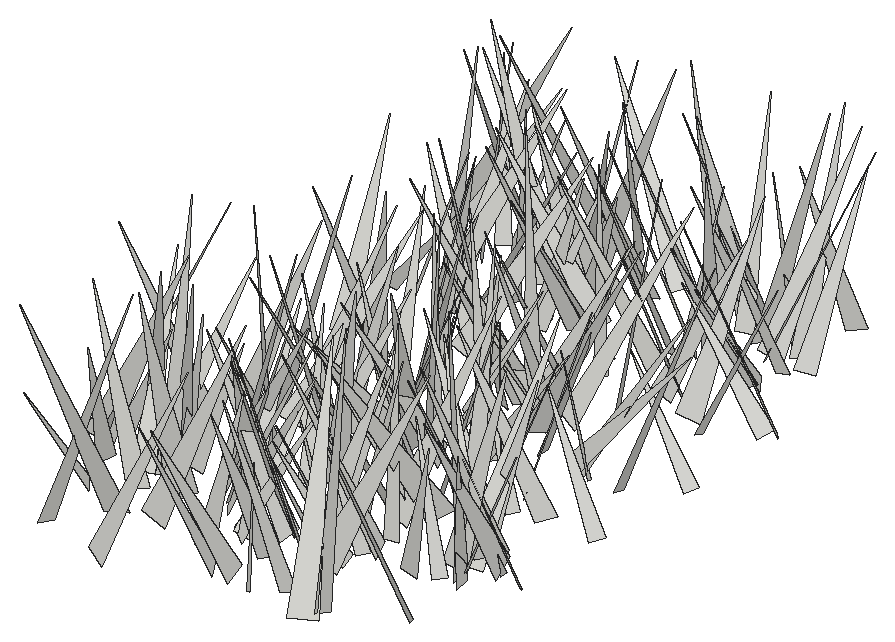
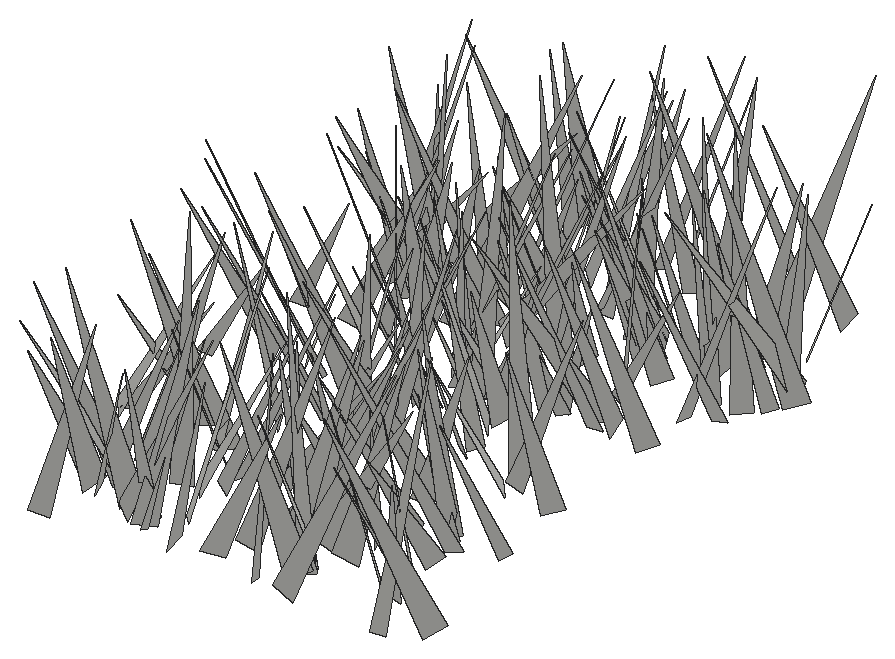
# SketchUp Ruby script. Lengths in inches.
U = 1.inch
M = Sketchup.active_model
def pt(a) = Geom::Point3d.new(a.map { |v| v * U })
def face(e, loops, mat)
  f = e.add_face(loops[0].map { |a| pt(a) })
  loops[1..].each { |l| e.add_face(l.map { |a| pt(a) }).erase! }
  f.material = f.back_material = mat if mat
  f
end
# faces: each face lists its corners as indices into pts; further lists are holes
def faces(e, pts, list, mat = nil) = list.each { |f| face(e, (f[0].is_a?(Array) ? f : [f]).map { |l| l.map { |i| pts[i] } }, mat) }
# xy, xz, yz: faces in a plane at the given z, y or x. An outline is a flat list of corners, or four numbers for a rectangle; further outlines are holes
def ring(l) = l.size == 4 ? [[l[0], l[1]], [l[2], l[1]], [l[2], l[3]], [l[0], l[3]]] : l.each_slice(2).to_a
def flat(e, list, mat, &to3) = list.each { |f| face(e, (f[0].is_a?(Array) ? f : [f]).map { |l| ring(l).map { |u, v| to3.(u, v) } }, mat) }
def xy(e, z, list, mat = nil) = flat(e, list, mat) { |x, y| [x, y, z] }
def xz(e, y, list, mat = nil) = flat(e, list, mat) { |x, z| [x, y, z] }
def yz(e, x, list, mat = nil) = flat(e, list, mat) { |y, z| [x, y, z] }
def lines(e, pts, list) = list.each { |a, b| e.add_line(pt(pts[a]), pt(pts[b])) }
# prism: a flat outline (further loops are holes) pulled along v
def prism(e, loops, v, mat = nil)
  f = face(e, loops, mat); d = Geom::Vector3d.new(v.map { |x| x * U })
  f.pushpull(f.normal.samedirection?(d) ? d.length : -d.length)
end
def box(e, o, s, mat = nil) = prism(e, [[o, [o[0] + s[0], o[1], o[2]], [o[0] + s[0], o[1] + s[1], o[2]], [o[0], o[1] + s[1], o[2]]]], [0, 0, s[2]], mat)
def at(x, y, z, deg = 0) = Geom::Transformation.translation(pt([x, y, z])) * Geom::Transformation.rotation(ORIGIN, Z_AXIS, deg.degrees)
def axes(o, x, y, z) = Geom::Transformation.new([*x, 0, *y, 0, *z, 0, *pt(o).to_a, 1])
def part(name) = M.definitions.add(name)
# library, detail: a bought-in or finely detailed component or shape, given as its bounding box
def library(name, o, s) = part(name).tap { |d| box(d.entities, o, s) }
def detail(e, o, s) = box(e.add_group.entities, o, s)
def put(e, d, t, mat = nil) = e.add_instance(d, t).tap { |i| i.material = mat if mat }
def group(e, t, mat = nil) = e.add_group.tap { |g| g.transformation = t; g.material = mat if mat }.entities
root = M.entities
c1 = part("fur_instance\#9")
p = [[0.8125,0,1.79],[0.67,-0.02,1.48],[0,-0.11,0],[0,0.11,0]]
faces(c1.entities,p,[[0,1,2,3]])
put(root,c1,axes([503.06,326.87,-21.66],[-7.42684,-1.75978,1.28146],[-1.36577,7.3143,2.12899],[1.69519,-1.81689,7.32954]))
put(root,c1,axes([499.76,320.31,-21.66],[7.75154,3.11882,0.30174],[2.75499,-7.16733,3.30818],[-1.4927,2.96765,7.67264]))
put(root,c1,axes([503.06,353.38,-21.66],[-0.43332,5.55714,0.38235],[5.39105,0.32188,1.43136],[-1.40165,-0.47995,5.3871]))
put(root,c1,axes([501.88,317.15,-21.66],[-3.67716,-3.23058,0.06887],[-2.92053,3.36739,2.02339],[1.38271,-1.47883,4.45691]))
put(root,c1,axes([498.68,354.93,-21.66],[6.56364,-3.25708,1.01889],[-3.38805,-5.95385,2.79299],[0.40967,2.94467,6.77415]))
put(root,c1,axes([499.84,323.02,-21.66],[2.80159,-3.67069,0.58517],[-3.61323,-2.51742,1.50747],[0.87232,1.36159,4.36468]))
put(root,c1,axes([500.91,319.94,-21.66],[4.81338,-2.70132,0.36004],[-2.51999,-4.69011,-1.49931],[-1.0375,-1.14068,5.31205]))
put(root,c1,axes([501.11,357.13,-21.66],[-2.73458,-7.67612,0.26637],[-7.34259,2.69559,2.30041],[2.25392,-0.53168,7.81722]))
put(root,c1,axes([499.58,354.53,-21.66],[2.70061,4.81345,0.08968],[4.52857,-2.505,-1.92033],[1.63383,-1.01307,5.17446]))
put(root,c1,axes([502.14,339.91,-21.66],[-4.09876,5.0884,1.14662],[4.86258,4.25523,-1.50159],[1.8873,0.0873,6.359]))
put(root,c1,axes([503.48,320.0625,-21.66],[-5.02723,4.35262,0.08247],[4.19421,4.87628,-1.68986],[1.1665,1.22544,6.43138]))
put(root,c1,axes([499.05,321.61,-21.66],[3.50419,-7.42751,1.71848],[-7.22357,-2.63012,3.36199],[2.43745,2.88357,7.49295]))
put(root,c1,axes([504.45,318.45,-21.66],[0.94645,-5.69848,3.07489],[-6.04954,-1.88624,-1.63358],[-2.30884,2.60631,5.54074]))
put(root,c1,axes([503.11,351.3125,-21.66],[4.45887,4.52554,1.75159],[4.30275,-4.78695,1.41478],[-2.24387,-0.18639,6.19358]))
put(root,c1,axes([501.33,325.75,-21.66],[0.65579,5.75921,0.77226],[5.58682,-0.41126,-1.67728],[1.5976,-0.92592,5.54845]))
put(root,c1,axes([500.93,324.29,-21.66],[8.00988,-2.00577,0.3429],[-1.833,-7.71682,-2.32157],[-0.88363,-2.17404,7.92412]))
put(root,c1,axes([503.67,348.66,-21.66],[-4.95607,3.58078,0.35964],[3.00453,4.45388,-2.94106],[1.98095,2.2034,5.36049]))
put(root,c1,axes([504.77,320.7,-21.66],[-7.79963,1.89477,1.60693],[1.33324,7.65978,-2.56065],[2.09639,2.17814,7.60707]))
put(root,c1,axes([501.02,345.64,-21.66],[2.58418,-3.37784,0.00054],[-2.92311,-2.23595,2.1316],[1.69269,1.29557,3.68023]))
put(root,c1,axes([505.22,315.52,-21.66],[0.76231,-8.24421,0.75454],[-8.09051,-0.90251,-1.68715],[-1.75496,0.57958,8.10565]))
put(root,c1,axes([505.65,339.03,-21.66],[-0.4063,-5.76079,1.26429],[-5.69006,0.04941,-1.60344],[-1.5519,1.32705,5.54804]))
put(root,c1,axes([502.75,312.21,-21.66],[7.28027,0.47928,1.68125],[-0.05604,-7.13268,2.27604],[-1.74733,2.22571,6.93193]))
put(root,c1,axes([504.96,345.73,-21.66],[-7.30658,0.78889,2.52937],[0.00726,7.42557,-2.29501],[2.64953,2.15518,6.98151]))
put(root,c1,axes([502.5625,330.76,-21.66],[4.48664,-4.30175,1.96808],[-4.72578,-3.95369,2.13158],[0.21294,2.89338,5.83878]))
put(root,c1,axes([503.9375,323.51,-21.66],[-0.90647,-5.11686,1.80724],[-5.12934,1.40604,1.40817],[1.7715,1.45288,5.00209]))
put(root,c1,axes([507.96,351.57,-21.66],[-2.53782,7.33959,2.16761],[7.45924,1.86167,2.42953],[-1.71111,-2.77006,7.37615]))
put(root,c1,axes([502.8125,324.51,-21.66],[-1.84089,-7.99139,1.4242],[-7.16502,2.28604,3.56596],[3.81486,0.4373,7.3848]))
put(root,c1,axes([508.27,356.82,-21.66],[-1.35129,-7.71927,0.81651],[-7.46816,1.06686,-2.27338],[-2.11671,1.16382,7.49966]))
put(root,c1,axes([509.98,351.07,-21.66],[-2.8355,7.09509,0.7949],[6.33308,2.10473,3.80453],[-3.2961,-2.05963,6.62616]))
put(root,c1,axes([503.71,353.32,-21.66],[4.52674,3.32324,0.78926],[3.39525,-4.2348,-1.64226],[0.37301,-1.78348,5.37013]))
put(root,c1,axes([507.53,327.41,-21.66],[-0.92246,-4.02488,0.49642],[-3.83236,0.69867,-1.45667],[-1.32631,0.78053,3.86377]))
put(root,c1,axes([505.39,330.08,-21.66],[-6.44163,0.17845,3.84936],[-1.24896,6.99677,-2.4144],[3.64548,2.71245,5.9747]))
put(root,c1,axes([504.375,346.27,-21.66],[1.31964,-4.20384,0.49444],[-3.9297,-1.02429,1.77946],[1.57296,0.96785,4.03079]))
put(root,c1,axes([506.0625,339.5,-21.66],[4.52328,4.39752,0.22155],[4.10164,-4.32376,2.0806],[-1.60118,1.34692,5.95561]))
put(root,c1,axes([508.7,343.64,-21.66],[-2.86629,5.19134,1.30889],[5.27356,2.48156,1.70596],[-0.92348,-1.94182,5.67938]))
put(root,c1,axes([503.67,346.99,-21.66],[1.59933,7.72158,1.03232],[7.26868,-1.09996,-3.03359],[2.80263,-1.55359,7.2786]))
put(root,c1,axes([508.52,325.45,-21.66],[-6.74078,-2.87477,2.26806],[-3.46071,6.55422,-1.97791],[1.19661,2.76122,7.05622]))
put(root,c1,axes([507.77,348.74,-21.66],[-5.27031,-0.93158,1.82448],[-1.52104,5.15288,-1.7627],[1.37223,2.13373,5.05341]))
put(root,c1,axes([504.91,345.66,-21.66],[1.45023,-6.39796,1.08768],[-6.25164,-1.07813,1.99368],[1.74182,1.45734,6.24998]))
put(root,c1,axes([505.53,322.18,-21.66],[1.80806,-4.3936,1.6396],[-4.55829,-1.23367,1.72079],[1.10181,2.10605,4.4285]))
put(root,c1,axes([507.14,319.12,-21.66],[6.25935,-4.83068,2.00086],[-4.50057,-6.56633,-1.77386],[-2.66155,-0.25726,7.70509]))
put(root,c1,axes([509.26,330.21,-21.66],[-0.23432,4.6061,1.3303],[4.44797,-0.2882,1.78136],[-1.78924,-1.31967,4.25416]))
put(root,c1,axes([506.16,337.6,-21.66],[2.3597,-7.64104,0.82634],[-7.58316,-2.17409,1.55097],[1.25061,1.23463,7.84527]))
put(root,c1,axes([506.36,330.87,-21.66],[2.2285,7.10603,0.93052],[7.02267,-1.97084,-1.76797],[1.42959,-1.39565,7.23438]))
put(root,c1,axes([507.85,322.89,-21.66],[6.46332,2.41268,1.62775],[2.03661,-6.58136,1.66821],[-2.07914,1.05343,6.69422]))
put(root,c1,axes([506.77,346.41,-21.66],[5.85572,0.96623,0.0245],[0.91904,-5.61274,1.69591],[-0.29926,1.66948,5.68743]))
put(root,c1,axes([506.53,329.82,-21.66],[-2.61013,7.00123,1.33294],[6.01827,2.92557,-3.58165],[3.81765,0.17478,6.55758]))
put(root,c1,axes([509.18,352.67,-21.66],[4.35483,5.04158,0.80125],[4.65214,-4.35304,2.10539],[-2.1017,0.81089,6.32055]))
put(root,c1,axes([509.52,321.8,-21.66],[-3.94963,4.34285,0.40783],[4.0226,3.83915,-1.92507],[1.68683,1.01332,5.54563]))
put(root,c1,axes([509.48,320.42,-21.66],[4.83042,2.64277,1.00625],[2.0268,-4.62442,2.4159],[-1.97202,1.72053,4.9478]))
put(root,c1,axes([510.93,333.45,-21.66],[-5.92228,3.52878,0.304],[3.26745,5.67188,-2.1844],[1.36692,1.73077,6.53866]))
put(root,c1,axes([506.74,324.27,-21.66],[3.69144,-5.31541,0.62902],[-5.0613,-3.21782,2.51095],[1.74141,1.9152,5.96452]))
put(root,c1,axes([510.52,337.67,-21.66],[2.07794,4.44656,0.23399],[4.16362,-2.03187,1.63715],[-1.57826,0.49406,4.62704]))
put(root,c1,axes([511.91,349.7,-21.66],[2.26565,-5.57265,3.25786],[-5.77256,-3.29433,-1.62055],[-2.88887,2.21229,5.79322]))
put(root,c1,axes([511.16,352.59,-21.66],[3.93068,-5.30389,1.53813],[-4.85639,-4.21869,-2.1367],[-2.62918,-0.13704,6.24628]))
put(root,c1,axes([507.51,310.72,-21.66],[3.41975,6.53108,1.33927],[6.45057,-2.86091,-2.51965],[1.68487,-2.30293,6.92828]))
put(root,c1,axes([513.34,349.39,-21.66],[-6.69596,1.51903,0.23584],[1.52209,6.40398,1.96756],[-0.2152,-1.96993,6.57815]))
put(root,c1,axes([511.57,324.86,-21.66],[-4.67511,2.29396,0.21165],[2.12082,4.47274,-1.63107],[0.89953,1.37696,4.94555]))
put(root,c1,axes([507.37,316.18,-21.66],[1.82991,-7.19945,3.13467],[-7.38413,-0.48301,3.20126],[2.67073,3.59742,6.70317]))
put(root,c1,axes([512.45,348.3,-21.66],[-0.7364,-6.55979,0.93298],[-6.36781,0.44127,-1.92351],[-1.83094,1.10364,6.31453]))
put(root,c1,axes([509.65,330.82,-21.66],[-4.5359,3.17744,2.60533],[2.766,5.23085,-1.56386],[3.0386,-0.01843,5.3127]))
put(root,c1,axes([512.42,331.92,-21.66],[-0.71726,5.0627,1.58469],[5.02661,0.13746,1.836],[-1.69568,-1.73401,4.77227]))
put(root,c1,axes([508.78,330.66,-21.66],[0.50211,5.33526,1.29674],[5.04367,0.06639,-2.22613],[2.16978,-1.38897,4.87457]))
put(root,c1,axes([509.16,319.67,-21.66],[3.22787,2.03353,0.24614],[1.96333,-2.94045,-1.45397],[0.58408,-1.35405,3.52709]))
put(root,c1,axes([514.18,355.79,-21.66],[-4.44973,5.42889,0.1833],[5.21151,4.19987,2.12315],[-1.53186,-1.48148,6.69068]))
put(root,c1,axes([508.75,354.73,-21.66],[6.76451,-3.26106,1.25254],[-3.47694,-6.54929,1.72622],[-0.33809,2.1058,7.30844]))
put(root,c1,axes([510.46,356.64,-21.66],[5.99792,1.55177,2.60045],[2.40829,-5.94226,-2.00876],[-1.83589,-2.72525,5.86071]))
put(root,c1,axes([509.88,348.4,-21.66],[-0.77614,4.62516,2.62163],[4.88719,1.66369,-1.48826],[2.09294,-2.16967,4.44742]))
put(root,c1,axes([510.63,347.02,-21.66],[-3.36626,3.2291,1.55087],[2.48228,3.63709,-2.18492],[2.58275,0.71309,4.12128]))
put(root,c1,axes([508.62,354.16,-21.66],[8.12463,-0.31909,0.21051],[-0.21684,-7.53553,-3.0536],[-0.31483,-3.04462,7.53571]))
put(root,c1,axes([511.35,334.3,-21.66],[6.37842,4.90538,1.53696],[4.59516,-6.53882,1.79932],[-2.30422,0.53885,7.84279]))
put(root,c1,axes([513.98,325.45,-21.66],[-4.11377,-6.51171,1.45116],[-6.65439,3.88319,-1.43913],[-0.47668,1.98739,7.56666]))
put(root,c1,axes([513.31,353.8,-21.66],[0.28426,-7.43419,0.75555],[-7.30944,-0.43371,-1.51752],[-1.55247,0.68085,7.28321]))
put(root,c1,axes([509.05,342.15,-21.66],[-0.59602,7.49567,1.64856],[6.68012,1.32078,-3.59019],[3.77872,-1.15261,6.60687]))
put(root,c1,axes([514.71,338.86,-21.66],[-5.12266,-6.1706,2.10185],[-6.50165,4.64284,-2.21548],[-0.47189,3.01719,7.70776]))
put(root,c1,axes([509.48,322.7,-21.66],[2.07826,-5.21506,0.82935],[-4.82149,-1.51054,2.58366],[2.15357,1.65083,4.98405]))
put(root,c1,axes([510.92,321.26,-21.66],[6.38764,-4.10189,0.26345],[-3.90919,-6.21298,-1.95294],[-1.27011,-1.50671,7.33577]))
put(root,c1,axes([514.6,319.49,-21.66],[-6.87538,0.87455,0.95023],[1.06547,6.75006,1.49673],[0.72976,-1.61573,6.76724]))
put(root,c1,axes([517.27,325.55,-21.66],[-4.42248,-6.55022,0.11235],[-5.68971,3.77318,-3.9833],[-3.24733,2.30957,6.8262]))
put(root,c1,axes([513.23,332.02,-21.66],[-6.54697,-3.05595,0.68846],[-2.14459,5.53525,4.1758],[2.28332,-3.56338,5.89613]))
put(root,c1,axes([509.73,320.07,-21.66],[5.9079,4.20697,0.32991],[4.15488,-5.69984,-1.72033],[0.73785,-1.5887,7.04573]))
put(root,c1,axes([510.15,336.9375,-21.66],[7.393,0.04175,0.28729],[0.1077,-7.1937,-1.72622],[-0.26959,-1.72907,7.18877]))
put(root,c1,axes([513.57,313.9375,-21.66],[-5.24067,-3.21189,0.67738],[-2.84495,5.08085,2.08111],[1.63749,-1.45206,5.78359]))
put(root,c1,axes([516.1,346.87,-21.66],[-2.43401,-4.94438,0.27236],[-4.40728,2.02468,-2.63096],[-2.25763,1.37813,4.84245]))
put(root,c1,axes([511,350.95,-21.66],[2.55159,-4.81811,0.15811],[-4.66384,-2.42197,1.46026],[1.21971,0.81832,5.25284]))
put(root,c1,axes([515.98,339.98,-21.66],[-8.04638,-2.10125,0.20494],[-2.02323,7.90531,1.61682],[0.60315,-1.51404,8.15753]))
put(root,c1,axes([512.46,331.36,-21.66],[4.4552,2.25801,0.37031],[2.04407,-4.29173,1.57715],[-1.02836,1.2518,4.7392]))
put(root,c1,axes([512.44,317.85,-21.66],[-0.90144,4.87523,0.09791],[4.65666,0.89022,-1.45364],[1.44671,0.1723,4.73998]))
put(root,c1,axes([515.92,329.59,-21.66],[-4.47703,-2.46915,0.00102],[-2.34184,4.24552,-1.62229],[-0.78262,1.42103,4.84857]))
put(root,c1,axes([511.85,315.14,-21.66],[0.68635,-5.64905,2.27441],[-5.90756,-0.06201,1.6287],[1.47832,2.3749,5.45254]))
put(root,c1,axes([513.93,332.74,-21.66],[3.59429,3.23742,0.8797],[2.57384,-3.488,2.32011],[-2.15177,1.23558,4.24464]))
put(root,c1,axes([515.55,331.71,-21.66],[1.80048,6.74236,1.9451],[6.61582,-2.30046,1.85022],[-2.33959,-1.31645,6.72888]))
put(root,c1,axes([515.43,339.6875,-21.66],[1.43774,-5.64122,0.58152],[-5.34924,-1.54822,-1.79367],[-1.88339,0.09091,5.53834]))
put(root,c1,axes([514.48,331.58,-21.66],[3.32895,2.2471,0.95718],[1.81279,-3.35751,1.57751],[-1.63691,0.85163,3.69362]))
put(root,c1,axes([514.99,314.05,-21.66],[-6.3203,-1.31951,1.76492],[-0.3807,5.93404,3.07318],[2.17051,-2.80147,5.67828]))
put(root,c1,axes([513.97,320.22,-21.66],[-3.49524,-7.20934,0.56433],[-6.86604,3.50524,2.25399],[2.26947,-0.49846,7.68835]))
put(root,c1,axes([516.67,356.22,-21.66],[-7.00273,-0.39667,0.95685],[-0.59042,6.90153,-1.45992],[0.85107,1.52402,6.86034]))
put(root,c1,axes([516.31,339.62,-21.66],[1.43872,7.93621,2.15807],[7.82752,-1.99366,2.11323],[-2.52399,-1.65906,7.7838]))
put(root,c1,axes([515.67,332.08,-21.66],[-6.83742,-2.67371,1.15288],[-1.91772,6.34944,3.35188],[2.19094,-2.7864,6.53176]))
put(root,c1,axes([515.23,316.875,-21.66],[2.94915,-5.28887,0.70098],[-5.06545,-3.02722,-1.5291],[-1.67475,-0.15728,5.85931]))
put(root,c1,axes([512.29,317.73,-21.66],[3.25743,4.86298,0.41292],[4.6269,-2.91916,-2.12138],[1.55271,-1.50328,5.4552]))
put(root,c1,axes([517.1875,341.92,-21.66],[-2.08811,-4.65792,0.59921],[-4.45757,1.75934,-1.85749],[-1.47829,1.27435,4.7546]))
put(root,c1,axes([517.51,317.51,-21.66],[-4.9951,-5.23204,0.99068],[-5.30492,4.77148,-1.54841],[-0.46216,1.77916,7.06595]))
put(root,c1,axes([513.07,325.55,-21.66],[1.49707,-8.01218,1.60299],[-8.01526,-1.12338,1.87068],[1.58751,1.88383,7.93327]))
put(root,c1,axes([515.04,340.98,-21.66],[3.98276,-1.20965,1.22676],[-0.42908,-3.68899,-2.24451],[-1.66855,-1.93873,3.5054]))
put(root,c1,axes([516.61,320.63,-21.66],[0.00954,3.59248,1.3323],[3.47361,-0.5704,1.51319],[-1.6171,-1.20405,3.25826]))
put(root,c1,axes([516.89,344.97,-21.66],[-6.05954,0.33778,0.89505],[0.02694,5.79744,-2.00555],[0.95629,1.97708,5.728]))
put(root,c1,axes([516.06,330.125,-21.66],[-6.64988,-1.58039,2.79885],[-2.32051,6.81074,-1.66765],[2.22405,2.38079,6.62853]))
put(root,c1,axes([516.16,334.47,-21.66],[-5.21181,1.32812,1.31914],[0.83689,5.14396,-1.87252],[1.67442,1.56295,5.04188]))
put(root,c1,axes([513.8125,332.01,-21.66],[7.80685,-2.34529,0.78759],[-1.91376,-7.37702,-2.99744],[-1.56786,-2.67335,7.58041]))
put(root,c1,axes([518.03,333.23,-21.66],[-7.28792,0.99409,0.70676],[0.80322,7.1337,-1.75122],[0.9179,1.65037,7.1439]))
put(root,c1,axes([516.79,313.05,-21.66],[1.83922,3.08635,0.93557],[2.6886,-2.06216,1.51739],[-1.78108,0.07419,3.25666]))
put(root,c1,axes([513.81,336.57,-21.66],[2.98745,4.37857,0.43851],[4.21633,-2.69647,-1.80015],[1.25963,-1.35874,4.98559]))
put(root,c1,axes([515.64,321.86,-21.66],[-3.26721,-5.06008,0.08616],[-4.54982,2.98181,2.58736],[2.21606,-1.33826,5.43917]))
put(root,c1,axes([518.59,349.45,-21.66],[-2.94744,-5.34651,0.76174],[-5.29498,2.69026,-1.60576],[-1.06233,1.42484,5.89017]))
put(root,c1,axes([518.61,314.4,-21.66],[-0.87207,-5.64239,2.10409],[-5.67136,0.05471,-2.20385],[-2.02471,2.277,5.26688]))
put(root,c1,axes([518.5,347.89,-21.66],[-6.87561,-0.89332,0.66489],[-0.69538,6.69239,1.80069],[0.86979,-1.71115,6.69549]))
put(root,c1,axes([517.01,340.14,-21.66],[-6.19203,-3.31038,1.54754],[-2.85802,6.28451,2.00782],[2.2771,-1.114,6.72819]))
put(root,c1,axes([519.61,350.22,-21.66],[-5.18196,-4.15409,0.26027],[-4.02731,4.89921,-1.98883],[-1.05116,1.70828,6.3367]))
put(root,c1,axes([516.36,321.3,-21.66],[-3.94538,2.89092,1.6801],[2.22143,4.20848,-2.02488],[2.49909,0.82308,4.45234]))
put(root,c1,axes([514.875,334.2,-21.66],[3.37481,3.69249,0.11879],[3.55193,-3.19874,-1.47981],[1.01606,-1.08238,4.77849]))
put(root,c1,axes([518.82,326.33,-21.66],[-6.06549,-1.51995,0.44377],[-1.27134,5.72216,2.22212],[0.94386,-2.06007,5.84487]))
put(root,c1,axes([517.81,353.55,-21.66],[-5.57338,-5.53642,0.81265],[-5.27737,5.58191,1.83481],[1.86058,-0.75178,7.63858]))
put(root,c1,axes([514.91,342.49,-21.66],[2.90433,5.023,0.38727],[4.82562,-2.64532,-1.87916],[1.44702,-1.25991,5.48948]))
put(root,c1,axes([520.38,329.62,-21.66],[-2.56552,5.11443,0.44811],[4.78646,2.20153,2.27666],[-1.85689,-1.39139,5.24939]))
put(root,c1,axes([519.24,320.43,-21.66],[-1.9475,3.70978,1.3462],[3.85912,1.47603,1.51527],[-0.82582,-1.85103,3.9063]))
put(root,c1,axes([519.05,319.28,-21.66],[-4.78281,-0.5343,0.54387],[-0.29464,4.48183,1.81189],[0.70318,-1.75621,4.45846]))
put(root,c1,axes([516.04,320.67,-21.66],[0.11042,6.13884,2.00494],[6.14565,0.51615,-1.91884],[1.98398,-1.94051,5.83229]))
put(root,c1,axes([519.72,321.39,-21.66],[-6.83596,-2.73328,0.53057],[-2.58478,6.75268,1.48423],[1.035,-1.18879,7.21098]))
put(root,c1,axes([517.64,321.875,-21.66],[5.12063,-0.00436,1.95562],[-0.62511,-5.19742,1.62522],[-1.85303,1.74129,4.85588]))
put(root,c1,axes([518.68,317.98,-21.66],[-3.83157,-3.11067,0.41222],[-2.87249,3.73899,1.51524],[1.26294,-0.9332,4.69694]))
put(root,c1,axes([519.47,322.68,-21.66],[1.15539,6.15443,1.22459],[6.01284,-1.44203,1.57415],[-1.79512,-0.86897,6.06086]))
put(root,c1,axes([521.3,355.08,-21.66],[-4.03956,-5.75099,0.92293],[-5.66396,3.6166,-2.25467],[-1.3584,2.0224,6.65646]))
put(root,c1,axes([519.375,355.58,-21.66],[4.80769,-4.80499,2.60276],[-4.52111,-5.44469,-1.70033],[-3.0695,0.49361,6.58109]))
put(root,c1,axes([520.01,326.58,-21.66],[4.91107,-6.51993,1.1851],[-5.42781,-4.80392,-3.93621],[-3.80168,-1.5638,7.15082]))
put(root,c1,axes([519.07,355.93,-21.66],[-5.21619,-2.22313,1.39253],[-1.54183,5.10575,2.37575],[2.12232,-1.75473,5.14847]))
put(root,c1,axes([520.09,354.01,-21.66],[0.51601,7.02264,0.2402],[6.84431,-0.55684,1.57697],[-1.5908,-0.11784,6.86272]))
put(root,c1,axes([521.15,327.85,-21.66],[-7.41355,2.38035,1.13819],[1.92535,7.2016,-2.52036],[1.80404,2.09598,7.36713]))
put(root,c1,axes([519.4375,326.76,-21.66],[5.08694,2.79276,1.06084],[2.31416,-5.00849,2.08845],[-1.88933,1.38471,5.41433]))
put(root,c1,axes([521.26,312.41,-21.66],[-6.0602,5.67803,0.65626],[5.53411,6.06799,-1.39639],[1.4298,0.57987,8.18634]))
put(root,c1,axes([521.66,313.7,-21.66],[-7.99125,0.08509,2.25297],[-0.74491,7.73167,-2.93422],[2.12796,3.02611,7.43355]))
put(root,c1,axes([518.09,324.85,-21.66],[1.6055,7.88479,1.47704],[7.72527,-1.11383,-2.45126],[2.16141,-1.87581,7.66412]))
put(root,c1,axes([521.01,346.48,-21.66],[3.09687,5.17866,0.3937],[4.90573,-3.06729,1.75775],[-1.70508,0.58082,5.7723]))
put(root,c1,axes([522.91,329.43,-21.66],[-0.96186,4.58475,0.31518],[4.19254,0.74357,1.97843],[-1.88199,-0.68675,4.24628]))
put(root,c1,axes([520.75,341.45,-21.66],[6.22186,3.72093,2.03459],[3.43335,-6.54009,1.46143],[-2.48938,0.27987,7.10078]))
put(root,c1,axes([519.85,336,-21.66],[6.47636,2.00005,0.90058],[1.74291,-6.39683,1.67254],[-1.33173,1.35459,6.56857]))
put(root,c1,axes([517.88,337.52,-21.66],[7.15691,-3.14413,0.26361],[-3.09126,-6.8566,2.14652],[0.63178,2.06831,7.5166]))
put(root,c1,axes([518.65,339.72,-21.66],[2.72489,7.5123,0.23605],[7.26372,-2.56761,-2.13568],[1.931,-0.94238,7.70056]))
put(root,c1,axes([518.34,318.03,-21.66],[2.77972,-6.83526,2.99642],[-7.05556,-1.36449,3.4327],[2.43278,3.85274,6.53179]))
put(root,c1,axes([524.1,324.5,-21.66],[-2.5947,5.83184,0.30944],[5.66182,2.42897,1.69778],[-1.43174,-0.96349,6.15308]))
put(root,c1,axes([521.63,346.25,-21.66],[-2.90473,-5.90083,0.221],[-5.68544,2.86131,1.67173],[1.5951,-0.54696,6.36102]))
put(root,c1,axes([521.09,330.61,-21.66],[-4.22534,-4.50008,2.6097],[-4.33201,4.90527,1.44456],[2.88009,0.77613,6.00146]))
put(root,c1,axes([520.625,350.59,-21.66],[0.39282,-7.92697,1.06347],[-7.86049,-0.18606,1.51663],[1.47665,1.11832,7.79044]))
put(root,c1,axes([523.93,335.14,-21.66],[-3.59352,-1.36236,0.30323],[-1.35819,3.22059,-1.62619],[-0.32136,1.6227,3.48208]))
put(root,c1,axes([526.19,316.1,-21.66],[-4.35257,-4.39527,0.35538],[-3.69396,3.36161,-3.66659],[-2.40819,2.78761,4.98191]))
put(root,c1,axes([524.03,353.92,-21.66],[-5.16392,-1.1559,0.80889],[-1.35151,4.93357,-1.57791],[0.40477,1.72635,5.05098]))
put(root,c1,axes([524.86,330.07,-21.66],[-3.6368,4.97548,2.15784],[5.29036,2.68314,2.72961],[-1.1932,-3.26854,5.52548]))
put(root,c1,axes([517.91,332.21,-21.66],[5.88193,4.68919,0.48239],[4.10623,-4.71789,-4.20698],[2.31519,-3.54559,6.23594]))
put(root,c1,axes([524.42,320.9375,-21.66],[-1.36293,4.52681,0.55653],[4.38086,1.13777,1.47406],[-1.26877,-0.93423,4.49185]))
put(root,c1,axes([522.22,331.36,-21.66],[4.78963,3.34115,0.62659],[3.09789,-4.73577,1.57225],[-1.39963,0.95165,5.62422]))
put(root,c1,axes([526.97,323.58,-21.66],[-3.79929,-4.93063,0.76728],[-4.2284,2.66909,-3.78564],[-2.64961,2.81057,4.94112]))
put(root,c1,axes([521.625,353.9,-21.66],[7.44072,-1.6859,2.03296],[-2.09272,-7.4711,1.46382],[-1.61112,1.91833,7.48758]))
put(root,c1,axes([524.76,351.7,-21.66],[-0.6126,-5.21006,0.97224],[-5.10965,0.32064,-1.50131],[-1.40764,1.1035,5.02654]))
put(root,c1,axes([524.51,353.7,-21.66],[-6.77077,3.15469,0.89527],[2.64884,6.47215,-2.77341],[1.93319,2.18084,6.93567]))
put(root,c1,axes([520.92,345.4375,-21.66],[0.63179,6.0642,2.01169],[5.81387,0.29266,-2.70812],[2.6496,-2.08816,5.46258]))
put(root,c1,axes([524.2,349.03,-21.66],[4.00993,-5.51552,0.33203],[-5.14979,-3.87921,-2.24547],[-2.00271,-1.06842,6.43882]))
put(root,c1,axes([524.9,358.26,-21.66],[2.07945,-5.56592,1.40736],[-5.43571,-2.39045,-1.42237],[-1.84751,0.76846,5.76892]))
put(root,c1,axes([522.63,320.32,-21.66],[0.54307,-5.39112,1.14857],[-5.29865,-0.1925,1.60174],[1.51911,1.25582,5.17624]))
put(root,c1,axes([525.84,321.13,-21.66],[-7.59721,-1.99805,2.32928],[-2.54922,7.5713,-1.81993],[1.70857,2.41215,7.64184]))
put(root,c1,axes([524.49,349.97,-21.66],[-4.06772,-3.26977,0.32403],[-2.78571,3.7053,2.41936],[1.74246,-1.70943,4.62433]))
put(root,c1,axes([522.48,326.83,-21.66],[4.18709,2.7222,0.51054],[2.74144,-3.94162,-1.4666],[0.39441,-1.502,4.77401]))
put(root,c1,axes([522.96,352.81,-21.66],[-0.55252,7.61083,1.2014],[7.43516,0.84266,-1.91879],[2.02152,-1.01911,7.38568]))
put(root,c1,axes([522.96,352.45,-21.66],[6.18332,3.30926,0.01495],[3.17233,-5.93637,1.96995],[-0.9422,1.73008,6.73082]))
put(root,c1,axes([525.93,324.79,-21.66],[-7.13222,-2.21187,1.52983],[-1.72076,7.08542,2.22194],[2.06682,-1.73369,7.12909]))
put(root,c1,axes([525.35,323.9375,-21.66],[3.42862,-3.42654,1.21049],[-3.04602,-3.61734,-1.61199],[-1.98197,-0.36822,4.57144]))
put(root,c1,axes([523.85,344.22,-21.66],[-1.22058,7.14872,1.6543],[7.02907,1.62036,-1.81584],[2.10547,-1.26529,7.02116]))
put(root,c1,axes([524.87,322.98,-21.66],[-5.0261,5.87636,0.71878],[5.2638,4.86732,-2.98524],[2.70938,1.44485,7.13314]))
put(root,c1,axes([525.7,352.55,-21.66],[-4.59878,4.14257,0.47856],[3.69105,4.37512,-2.40275],[1.94062,1.49539,5.70408]))
put(root,c1,axes([525.05,322.54,-21.66],[5.40862,3.75774,0.29196],[3.28966,-4.95573,2.84217],[-1.83956,2.18614,5.94103]))
put(root,c1,axes([524.01,325.41,-21.66],[3.16186,-4.77933,2.12939],[-5.21892,-2.70344,1.68164],[0.37303,2.68757,5.47827]))
put(root,c1,axes([528.46,345.53,-21.66],[-4.24155,2.82864,0.08548],[2.61337,3.85608,2.07369],[-1.08573,-1.76881,4.65744]))
put(root,c1,axes([529.08,345.83,-21.66],[-5.24888,-4.54366,0.15791],[-4.36596,4.97023,-2.11085],[-1.26815,1.69482,6.61361]))
put(root,c1,axes([524.28,322.48,-21.66],[1.86303,-6.4471,2.90273],[-6.99316,-1.23765,1.73947],[1.04242,3.21946,6.48153]))
put(root,c1,axes([525.15,321.9,-21.66],[5.21183,-0.69159,1.00189],[-0.40075,-5.13378,-1.45906],[-1.14955,-1.3458,5.051]))
put(root,c1,axes([528.57,330.04,-21.66],[-2.74524,3.88345,0.46197],[3.73915,2.44095,1.70042],[-1.14601,-1.33847,4.4414]))
put(root,c1,axes([528.73,322.93,-21.66],[-3.23089,-3.2407,0.20186],[-3.09319,2.98531,-1.58167],[-0.98745,1.25194,4.29408]))
put(root,c1,axes([525.39,343.25,-21.66],[4.79921,1.03907,0.41248],[0.79797,-4.45725,1.94381],[-0.78297,1.82633,4.50929]))
put(root,c1,axes([522.77,335.61,-21.66],[5.32286,5.30667,0.20638],[4.93366,-4.8331,-2.97258],[1.96528,-2.23975,6.90343]))
put(root,c1,axes([526.5,324.04,-21.66],[-6.90134,-2.30385,2.57209],[-0.73953,6.60101,3.92832],[3.37291,-3.26662,6.12409]))
put(root,c1,axes([522.13,335.68,-21.66],[4.7067,5.43888,0.18038],[4.50837,-3.76361,-4.15655],[3.04771,-2.83211,5.87006]))
put(root,c1,axes([529.1875,337.85,-21.66],[-2.95637,3.32548,0.26078],[3.10336,2.61427,1.84435],[-1.22309,-1.40488,4.04936]))
put(root,c1,axes([526.02,335.22,-21.66],[6.68377,2.4417,1.0502],[1.89436,-6.36953,2.75283],[-1.86446,2.28139,6.56175]))
